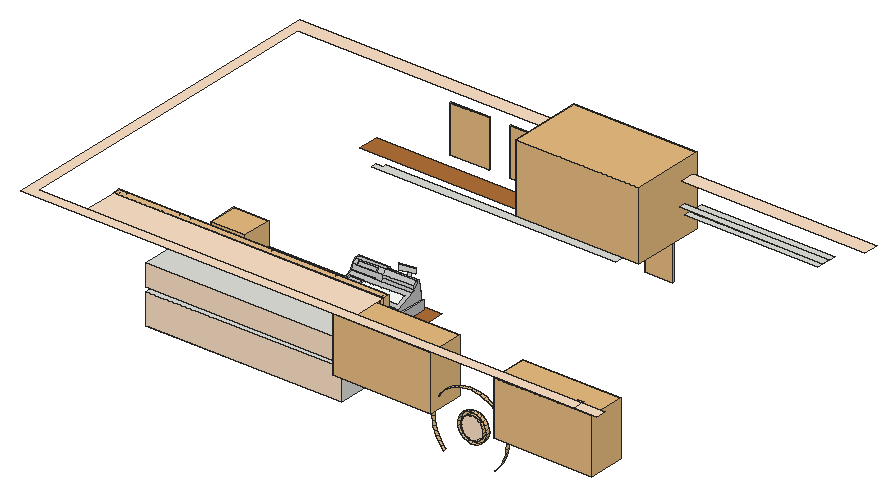
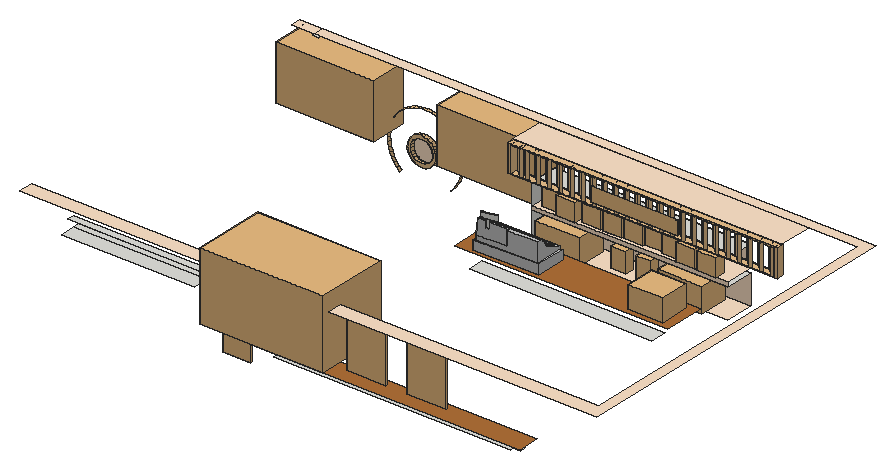
# SketchUp Ruby script. Lengths in inches.
U = 1.inch
M = Sketchup.active_model
def pt(a) = Geom::Point3d.new(a.map { |v| v * U })
def face(e, loops, mat)
  f = e.add_face(loops[0].map { |a| pt(a) })
  loops[1..].each { |l| e.add_face(l.map { |a| pt(a) }).erase! }
  f.material = f.back_material = mat if mat
  f
end
# faces: each face lists its corners as indices into pts; further lists are holes
def faces(e, pts, list, mat = nil) = list.each { |f| face(e, (f[0].is_a?(Array) ? f : [f]).map { |l| l.map { |i| pts[i] } }, mat) }
# xy, xz, yz: faces in a plane at the given z, y or x. An outline is a flat list of corners, or four numbers for a rectangle; further outlines are holes
def ring(l) = l.size == 4 ? [[l[0], l[1]], [l[2], l[1]], [l[2], l[3]], [l[0], l[3]]] : l.each_slice(2).to_a
def flat(e, list, mat, &to3) = list.each { |f| face(e, (f[0].is_a?(Array) ? f : [f]).map { |l| ring(l).map { |u, v| to3.(u, v) } }, mat) }
def xy(e, z, list, mat = nil) = flat(e, list, mat) { |x, y| [x, y, z] }
def xz(e, y, list, mat = nil) = flat(e, list, mat) { |x, z| [x, y, z] }
def yz(e, x, list, mat = nil) = flat(e, list, mat) { |y, z| [x, y, z] }
def lines(e, pts, list) = list.each { |a, b| e.add_line(pt(pts[a]), pt(pts[b])) }
# prism: a flat outline (further loops are holes) pulled along v
def prism(e, loops, v, mat = nil)
  f = face(e, loops, mat); d = Geom::Vector3d.new(v.map { |x| x * U })
  f.pushpull(f.normal.samedirection?(d) ? d.length : -d.length)
end
def box(e, o, s, mat = nil) = prism(e, [[o, [o[0] + s[0], o[1], o[2]], [o[0] + s[0], o[1] + s[1], o[2]], [o[0], o[1] + s[1], o[2]]]], [0, 0, s[2]], mat)
def at(x, y, z, deg = 0) = Geom::Transformation.translation(pt([x, y, z])) * Geom::Transformation.rotation(ORIGIN, Z_AXIS, deg.degrees)
def axes(o, x, y, z) = Geom::Transformation.new([*x, 0, *y, 0, *z, 0, *pt(o).to_a, 1])
def part(name) = M.definitions.add(name)
# library, detail: a bought-in or finely detailed component or shape, given as its bounding box
def library(name, o, s) = part(name).tap { |d| box(d.entities, o, s) }
def detail(e, o, s) = box(e.add_group.entities, o, s)
def put(e, d, t, mat = nil) = e.add_instance(d, t).tap { |i| i.material = mat if mat }
def group(e, t, mat = nil) = e.add_group.tap { |g| g.transformation = t; g.material = mat if mat }.entities
root = M.entities
M.materials.add("[Color C02]").color = [255, 228, 201]
M.materials.add("[Wood Bamboo]").color = [177, 112, 56]
M.materials.add("cash register keys").color = [249, 253, 248]
M.materials.add("ciber café cafeteira 2").color = [198, 198, 198]
M.materials.add("images").color = [235, 194, 141]
c1 = library("kitchen",[57.57,5.21,10.61],[18.31,18.31,13.72])
c2 = library("Group\#123",[0,0,0],[8.32,16.8,15.65])
c3 = library("Espresso+machine+low+poly",[-3.8125,0,0],[25.21,40.375,21.95])
c4 = library("Group\#75",[0,0,0],[34.67,0.75,41.45])
c5 = part("组\#40")
prism(c5.entities,[[[0,18.82,110.24],[218.9,18.82,110.24],[218.9,18.82,0],[0,18.82,0]],[[2.84,18.82,2.84],[216.06,18.82,2.84],[216.06,18.82,107.4],[2.84,18.82,107.4]]],[0,-18.82,0])
c6 = part("组\#36")
prism(c6.entities,[[[1.84,0,0],[0,0,0],[5.28,7.875,0],[7.11,7.875,0]]],[0,0,104.5625])
c7 = part("组\#49")
put(c7.entities,c5,at(0,1.23,0),"images")
put(c7.entities,c6,axes([8.22,1.23,2.84],[1.25286,0,0],[0,2.39,0],[0,0,1]),"images")
put(c7.entities,c6,axes([17.26,1.23,2.84],[1.25286,0,0],[0,2.39,0],[0,0,1]),"images")
put(c7.entities,c6,axes([26.3,1.23,2.84],[1.25286,0,0],[0,2.39,0],[0,0,1]),"images")
put(c7.entities,c6,axes([35.35,1.23,2.84],[1.25286,0,0],[0,2.39,0],[0,0,1]),"images")
put(c7.entities,c6,axes([71.52,1.23,2.84],[1.25286,0,0],[0,2.39,0],[0,0,1]),"images")
put(c7.entities,c6,axes([62.47,1.23,2.84],[1.25286,0,0],[0,2.39,0],[0,0,1]),"images")
put(c7.entities,c6,axes([44.39,1.23,2.84],[1.25286,0,0],[0,2.39,0],[0,0,1]),"images")
put(c7.entities,c6,axes([53.43,1.23,2.84],[1.25286,0,0],[0,2.39,0],[0,0,1]),"images")
put(c7.entities,c6,axes([89.6,1.23,2.84],[1.25286,0,0],[0,2.39,0],[0,0,1]),"images")
put(c7.entities,c6,axes([80.56,1.23,2.84],[1.25286,0,0],[0,2.39,0],[0,0,1]),"images")
put(c7.entities,c6,axes([98.64,1.23,2.84],[1.25286,0,0],[0,2.39,0],[0,0,1]),"images")
put(c7.entities,c6,axes([107.69,1.23,2.84],[1.25286,0,0],[0,2.39,0],[0,0,1]),"images")
put(c7.entities,c6,axes([125.77,1.23,2.84],[1.25286,0,0],[0,2.39,0],[0,0,1]),"images")
put(c7.entities,c6,axes([143.85,1.23,2.84],[1.25286,0,0],[0,2.39,0],[0,0,1]),"images")
put(c7.entities,c6,axes([116.73,1.23,2.84],[1.25286,0,0],[0,2.39,0],[0,0,1]),"images")
put(c7.entities,c6,axes([134.8125,1.23,2.84],[1.25286,0,0],[0,2.39,0],[0,0,1]),"images")
put(c7.entities,c6,axes([180.02,1.23,2.84],[1.25286,0,0],[0,2.39,0],[0,0,1]),"images")
put(c7.entities,c6,axes([170.98,1.23,2.84],[1.25286,0,0],[0,2.39,0],[0,0,1]),"images")
put(c7.entities,c6,axes([152.9,1.23,2.84],[1.25286,0,0],[0,2.39,0],[0,0,1]),"images")
put(c7.entities,c6,axes([161.9375,1.23,2.84],[1.25286,0,0],[0,2.39,0],[0,0,1]),"images")
put(c7.entities,c6,axes([198.11,1.23,2.84],[1.25286,0,0],[0,2.39,0],[0,0,1]),"images")
put(c7.entities,c6,axes([189.07,1.23,2.84],[1.25286,0,0],[0,2.39,0],[0,0,1]),"images")
put(c7.entities,c6,axes([207.15,1.23,2.84],[1.25286,0,0],[0,2.39,0],[0,0,1]),"images")
put(c7.entities,c6,axes([3.02,1.23,2.84],[1.25286,0,0],[0,2.39,0],[0,0,1]),"images")
c8 = library("ME COFFCE",[24.16,0,0],[47.26,9.94,0.98])
c9 = library("Countertop blender",[-3.14,-3.14,0],[6.83,6.28,15])
c10 = part("Component\#80")
xy(c10.entities,0,[[4.632,0.029,4.499,0.032,4.417,0.044,4.351,0.06,4.27,0.071,4.201,0.069,4.158,0.068,4.114,0.081,4.08,0.096,4.058,0.095,4.037,0.097,4.036,0.106,4.019,0.112,3.989,0.137,3.907,0.15,3.851,0.172,3.794,0.2,3.729,0.203,3.682,0.236,3.678,0.265,3.623,0.28,3.603,0.307,3.598,0.343,3.568,0.367,3.529,0.378,3.516,0.396,3.507,0.423,3.511,0.432,3.533,0.433,3.574,0.441,3.616,0.451,3.62,0.461,3.608,0.47,3.587,0.469,3.565,0.471,3.547,0.486,3.546,0.495,3.537,0.562,3.538,0.589,3.589,0.609,3.579,0.646,3.514,0.649,3.375,0.645,3.369,0.654,3.389,0.659,3.403,0.676,3.44,0.684,3.438,0.693,3.42,0.708,3.408,0.717,3.387,0.717,3.365,0.721,3.363,0.732,3.367,0.742,3.517,0.746,3.538,0.751,3.516,0.753,3.495,0.752,3.486,0.779,3.497,0.819,3.504,0.84,3.526,0.841,3.54,0.857,3.528,0.866,3.506,0.866,3.441,0.873,3.397,0.876,3.373,0.894,3.309,0.897,3.261,0.893,3.262,0.884,3.259,0.866,3.238,0.865,3.083,0.856,3.035,0.855,3.008,0.852,3.01,0.843,3.014,0.81,3.027,0.792,3.071,0.789,3.08,0.759,3.04,0.705,3.038,0.638,3.019,0.621,3.032,0.603,3.047,0.576,3.014,0.54,2.974,0.519,2.841,0.478,2.675,0.437,2.623,0.431,2.62,0.412,2.613,0.385,2.616,0.366,2.617,0.355,2.596,0.352,2.528,0.343,2.51,0.285,2.445,0.254,2.376,0.252,2.205,0.247,2.168,0.21,2.132,0.202,2.11,0.201,2.053,0.19,1.984,0.189,1.955,0.201,1.979,0.218,2.018,0.244,2.061,0.278,2.112,0.3,2.26,0.308,2.267,0.336,2.266,0.345,2.286,0.35,2.301,0.358,2.315,0.376,2.276,0.384,2.267,0.412,2.265,0.421,2.286,0.424,2.334,0.425,2.348,0.442,2.347,0.451,2.36,0.472,2.39,0.486,2.454,0.488,2.439,0.515,2.421,0.531,2.398,0.537,2.355,0.543,2.335,0.563,2.285,0.578,2.254,0.644,2.248,0.683,2.182,0.693,2.126,0.712,2.061,0.712,2.007,0.718,1.977,0.735,1.989,0.763,1.98,0.828,1.916,0.859,1.855,0.871,1.846,0.928,1.782,0.964,1.711,0.971,1.708,0.99,1.664,0.995,1.588,1,1.432,0.996,1.405,0.995,1.407,0.986,1.408,0.977,1.386,0.948,1.391,0.911,1.341,0.889,1.325,0.821,1.33,0.784,1.308,0.756,1.253,0.731,1.246,0.701,1.193,0.633,1.181,0.607,1.145,0.595,1.083,0.581,0.919,0.563,0.876,0.562,0.894,0.555,0.897,0.535,0.918,0.535,0.94,0.531,0.942,0.522,0.923,0.506,0.867,0.486,0.848,0.469,0.827,0.466,0.829,0.455,0.835,0.418,0.87,0.403,0.867,0.384,0.83,0.351,0.816,0.335,0.818,0.326,0.823,0.291,0.826,0.271,0.828,0.26,0.808,0.254,0.744,0.253,0.573,0.248,0.488,0.246,0.425,0.237,0.341,0.196,0.294,0.19,0.298,0.162,0.303,0.131,0.287,0.103,0.194,0.082,0.131,0.073,0.061,0.078,0.013,0.077,0,0.094,0,0.215,0.054,0.209,0.124,0.23,0.173,0.258,0.203,0.264,0.218,0.266,0.221,0.273,0.249,0.292,0.279,0.299,0.322,0.32,0.363,0.33,0.38,0.34,0.378,0.387,0.4,0.399,0.434,0.393,0.463,0.402,0.514,0.423,0.56,0.425,0.566,0.438,0.569,0.466,0.563,0.49,0.59,0.48,0.621,0.481,0.687,0.483,0.767,0.49,0.774,0.517,0.769,0.552,0.767,0.565,0.776,0.577,0.807,0.605,0.85,0.626,0.895,0.639,0.893,0.652,0.89,0.667,0.9,0.679,0.951,0.7,0.966,0.726,1.029,0.751,1.059,0.757,1.069,0.769,1.067,0.782,1.084,0.794,1.106,0.807,1.104,0.82,1.094,0.88,1.092,0.894,1.058,0.895,1.113,0.908,1.175,0.909,1.222,0.911,1.224,0.924,1.227,0.953,1.245,0.963,1.28,0.964,1.272,0.993,1.231,1.007,1.232,1.02,1.231,1.029,1.246,1.032,1.277,1.037,1.343,1.039,1.354,1.044,1.345,1.05,1.317,1.055,1.295,1.073,1.293,1.086,1.277,1.113,1.22,1.14,1.231,1.159,1.231,1.195,1.484,1.207,1.592,1.192,1.643,1.172,1.703,1.165,1.792,1.138,1.84,1.137,1.864,1.121,1.922,1.089,2.01,1.068,2.021,1.028,2.104,1.005,2.192,0.984,2.245,0.952,2.308,0.917,2.33,0.877,2.413,0.852,2.471,0.821,2.476,0.783,2.544,0.758,2.58,0.725,2.618,0.675,2.744,0.708,2.739,0.745,2.769,0.757,2.767,0.776,2.735,0.793,2.805,0.85,2.85,0.833,2.914,0.838,2.988,0.881,3.03,0.892,3.049,0.911,3.09,0.921,3.089,0.93,3.089,0.967,3.146,0.985,3.191,1.007,3.22,1.034,3.234,1.05,3.207,1.081,3.261,1.105,3.284,1.08,3.37,1.08,3.383,1.061,3.404,1.062,3.496,1.065,3.538,1.073,3.536,1.082,3.512,1.1,3.491,1.102,3.465,1.131,3.372,1.149,3.433,1.171,3.499,1.16,3.52,1.163,3.599,1.177,3.663,1.183,3.6875,1.2,3.731,1.201,3.762,1.207,3.76,1.225,3.79,1.24,3.812,1.238,3.882,1.24,3.968,1.24,3.998,1.213,4.009,1.172,3.973,1.161,3.951,1.161,3.801,1.154,3.775,1.154,3.765,1.144,3.766,1.135,3.77,1.105,3.777,1.096,3.798,1.096,3.841,1.097,3.863,1.093,3.865,1.084,3.866,1.07,3.858,1.049,3.816,1.046,3.795,1.04,3.807,1.031,3.808,1.022,3.776,0.942,3.706,0.938,3.721,0.911,3.764,0.912,3.771,0.894,3.759,0.866,3.755,0.856,3.734,0.853,3.691,0.85,3.689,0.822,3.757,0.801,3.76,0.773,3.751,0.764,3.73,0.763,3.709,0.758,3.71,0.749,3.731,0.749,3.748,0.743,3.721,0.705,3.722,0.696,3.744,0.697,3.765,0.695,3.774,0.631,3.777,0.608,3.778,0.598,3.757,0.596,3.693,0.591,3.646,0.588,3.647,0.579,3.667,0.552,3.748,0.54,3.752,0.513,3.738,0.496,3.723,0.489,3.735,0.48,3.739,0.448,3.741,0.439,3.762,0.439,3.805,0.438,3.875,0.433,3.873,0.406,3.854,0.387,3.833,0.384,3.791,0.383,3.77,0.38,3.771,0.371,3.814,0.367,3.826,0.359,3.829,0.34,3.857,0.327,3.927,0.327,3.955,0.314,3.962,0.303,3.983,0.303,4.049,0.291,4.084,0.267,4.093,0.238,4.127,0.225,4.17,0.226,4.213,0.22,4.214,0.211,4.205,0.202,4.183,0.201,4.17,0.185,4.171,0.174,4.193,0.17,4.21,0.163,4.236,0.125,4.244,0.107,4.265,0.11,4.392,0.116,4.482,0.121,4.522,0.099,4.607,0.101,4.644,0.109,4.658,0.119,4.743,0.123,4.792,0.12,4.803,0.111,4.942,0.113,4.96,0.097,4.962,0.079,4.955,0.052,4.866,0.036,4.802,0.034],[7.489,0.131,7.472,0.169,7.381,0.18,7.377,0.199,7.376,0.209,7.353,0.211,7.309,0.209,7.251,0.188,7.144,0.235,7.104,0.241,7.082,0.24,7.037,0.239,6.97,0.244,6.939,0.263,6.891,0.285,6.888,0.304,6.875,0.323,6.852,0.322,6.807,0.326,6.797,0.354,6.778,0.37,6.733,0.374,6.726,0.383,6.723,0.402,6.721,0.455,6.717,0.483,6.721,0.493,6.743,0.493,6.787,0.497,6.786,0.507,6.785,0.516,6.762,0.518,6.727,0.529,6.725,0.538,6.723,0.557,6.714,0.617,6.706,0.672,6.713,0.701,6.75,0.712,6.794,0.72,6.792,0.73,6.806,0.749,6.837,0.767,6.86,0.768,6.868,0.785,6.849,0.801,6.826,0.803,6.782,0.801,6.718,0.817,6.699,0.833,6.703,0.843,6.725,0.846,6.747,0.851,6.783,0.867,6.787,0.92,6.771,0.95,6.746,0.967,6.677,0.979,6.627,0.978,6.493,0.974,6.465,0.971,6.467,0.961,6.468,0.952,6.471,0.93,6.423,0.912,6.426,0.893,6.398,0.858,6.348,0.852,6.304,0.848,6.305,0.839,6.308,0.82,6.305,0.769,6.29,0.718,6.293,0.699,6.277,0.691,6.233,0.685,6.238,0.657,6.245,0.647,6.267,0.648,6.312,0.647,6.314,0.637,6.316,0.618,6.314,0.596,6.293,0.591,6.271,0.586,6.272,0.576,6.28,0.526,6.272,0.471,6.166,0.43,6.055,0.424,6.0625,0.415,6.085,0.415,6.107,0.416,6.152,0.413,6.151,0.384,6.131,0.367,6.061,0.35,6.031,0.326,5.93,0.294,5.916,0.277,5.918,0.268,5.886,0.255,5.764,0.251,5.697,0.25,5.659,0.241,5.65,0.229,5.628,0.229,5.6,0.228,5.545,0.226,5.433,0.226,5.311,0.225,5.247,0.237,5.222,0.253,5.19,0.283,5.149,0.292,4.999,0.29,4.947,0.296,4.93,0.302,4.889,0.313,4.817,0.311,4.776,0.317,4.768,0.367,4.705,0.408,4.717,0.44,4.76,0.448,4.774,0.465,4.773,0.475,4.77,0.494,4.765,0.522,4.719,0.531,4.711,0.578,4.694,0.679,4.723,0.706,4.722,0.716,4.699,0.717,4.694,0.746,4.738,0.752,4.733,0.786,4.726,0.795,4.703,0.794,4.681,0.794,4.679,0.803,4.678,0.813,4.679,0.837,4.919,0.849,5.039,0.835,5.075,0.822,5.092,0.815,5.048,0.814,5.003,0.8125,4.962,0.79,4.948,0.772,4.95,0.763,4.912,0.752,4.89,0.749,4.892,0.74,4.896,0.711,4.898,0.701,4.921,0.7,4.993,0.702,5.038,0.703,5.06,0.703,5.073,0.694,5.059,0.677,5.001,0.656,4.89,0.646,4.868,0.645,4.869,0.636,4.874,0.607,4.982,0.596,4.979,0.545,5.01,0.529,5.073,0.521,5.081,0.474,5.056,0.454,5.046,0.444,5.024,0.443,4.979,0.442,4.957,0.442,4.938,0.42,4.952,0.372,4.96,0.353,5.045,0.351,5.156,0.354,5.191,0.341,5.193,0.331,5.195,0.322,5.218,0.317,5.249,0.333,5.307,0.349,5.424,0.352,5.501,0.328,5.545,0.329,5.567,0.329,5.598,0.349,5.64,0.365,5.706,0.369,5.818,0.372,5.855,0.38,5.851,0.411,5.836,0.43,5.814,0.432,5.816,0.451,5.858,0.505,5.959,0.539,5.952,0.584,5.949,0.608,5.972,0.635,6.016,0.641,6.039,0.642,6.03,0.661,6.027,0.68,6.026,0.689,5.981,0.69,5.958,0.69,5.951,0.699,5.95,0.709,5.948,0.718,6.014,0.727,6.018,0.737,5.973,0.743,5.964,0.764,5.982,0.794,5.956,0.848,6.057,0.854,6.095,0.862,6.124,0.889,6.172,0.903,6.149,0.907,6.105,0.906,6.04,0.923,6.013,1.031,6.003,1.055,5.991,1.064,6.041,1.068,6.164,1.071,6.253,1.071,6.3,1.063,6.321,1.035,6.322,1.025,6.351,1.023,6.434,1.026,6.569,1.029,6.692,1.033,6.742,1.034,6.772,1.062,7.018,1.068,7.114,1.064,7.159,1.065,7.163,1.036,7.142,0.987,7.149,0.939,7.105,0.928,7.083,0.925,7.069,0.906,7.02,0.856,7.001,0.839,7.005,0.81,7.012,0.76,6.99,0.718,6.98,0.67,6.983,0.649,6.985,0.639,6.97,0.622,6.939,0.607,6.927,0.578,6.935,0.556,6.953,0.55,6.945,0.528,6.924,0.482,6.939,0.379,7.004,0.35,7.007,0.331,7.009,0.322,7.039,0.306,7.171,0.281,7.315,0.283,7.338,0.283,7.35,0.274,7.354,0.245,7.394,0.239,7.466,0.244,7.585,0.266,7.626,0.258,7.644,0.249,7.651,0.239,7.679,0.238,7.898,0.265,8.014,0.269,8.064,0.27,8.092,0.271,8.114,0.271,8.119,0.281,8.112,0.328,8.11,0.347,8.089,0.378,8.058,0.396,8.043,0.424,8.036,0.474,8.031,0.515,7.975,0.554,7.967,0.613,8.004,0.67,8.119,0.687,8.117,0.706,8.115,0.716,8.12,0.726,8.147,0.726,8.263,0.742,8.307,0.748,8.359,0.773,8.403,0.779,8.426,0.78,8.436,0.79,8.473,0.803,8.539,0.809,8.648,0.834,8.668,0.854,8.738,0.872,8.776,0.888,8.859,0.89,8.993,0.896,9.124,0.878,9.175,0.877,9.218,0.847,9.27,0.832,9.315,0.833,9.346,0.848,9.413,0.85,9.525,0.853,9.57,0.852,9.633,0.84,9.635,0.82,9.569,0.811,9.453,0.799,9.409,0.797,9.462,0.77,9.503,0.759,9.571,0.754,9.593,0.754,9.605,0.745,9.608,0.726,9.696,0.69,9.698,0.671,9.673,0.644,9.629,0.638,9.627,0.609,9.684,0.606,9.717,0.607,9.739,0.607,9.735,0.598,9.663,0.546,9.641,0.54,9.643,0.531,9.665,0.531,9.673,0.512,9.569,0.495,9.57,0.443,9.555,0.423,9.49,0.407,9.44,0.406,9.418,0.405,9.396,0.407,9.391,0.397,9.394,0.378,9.466,0.38,9.488,0.381,9.495,0.371,9.442,0.346,9.332,0.334,9.318,0.316,9.316,0.288,9.311,0.238,9.303,0.222,9.28,0.221,9.203,0.219,9.076,0.211,8.826,0.204,8.743,0.201,8.698,0.203,8.685,0.212,8.655,0.23,8.627,0.232,8.582,0.23,8.51,0.228,8.47,0.234,8.468,0.244,8.454,0.263,8.432,0.262,8.388,0.261,8.138,0.252,8.143,0.223,8.091,0.198,7.983,0.176,7.937,0.153,7.865,0.151,7.748,0.148],[9.141,1.006,9.078,1.05,9.072,1.088,9.069,1.108,9.089,1.125,9.177,1.135,9.171,1.137,9.231,1.151,9.227,1.172,9.231,1.182,9.254,1.183,9.298,1.184,9.347,1.164,9.397,1.165,9.504,1.161,9.571,1.167,9.608,1.181,9.647,1.223,9.712,1.237,9.726,1.257,9.75,1.279,9.795,1.28,9.907,1.283,9.963,1.285,9.96,1.304,9.956,1.333,9.966,1.343,9.988,1.344,10.082,1.351,10.2,1.357,10.223,1.355,10.224,1.345,10.227,1.326,10.238,1.288,10.207,1.272,10.163,1.264,10.046,1.258,10.019,1.253,10.02,1.243,10.006,1.223,9.94,1.216,9.913,1.211,9.914,1.201,9.858,1.161,9.768,1.129,9.73,1.116,9.686,1.115,9.558,1.104,9.489,1.081,9.366,1.077,9.322,1.069,9.325,1.049,9.296,1.022,9.247,1.011],[4.831,1.075,4.757,1.083,4.65,1.119,4.613,1.135,4.625,1.167,4.627,1.186,4.662,1.214,4.673,1.216,4.762,1.221,4.878,1.237,4.9,1.237,4.91,1.247,4.982,1.254,5.105,1.257,5.163,1.252,5.182,1.235,5.185,1.216,5.253,1.215,5.293,1.209,5.326,1.181,5.282,1.175,5.259,1.174,5.221,1.166,5.222,1.125,5.197,1.105,5.125,1.098,5.009,1.085,4.876,1.077]])
p = [[0,0,0],[0,0.094,0]]
lines(c10.entities,p,[[0,1]])
c11 = part("PointCash_Register")
g1 = group(c11.entities,at(0,-0.25,0))
xy(g1,0,[[0,0.25,16,16.25]],"ciber café cafeteira 2")
xy(g1,4,[[[0,0.25,16,16.25],[0.5,0.75,15.5,15.75]]],"ciber café cafeteira 2")
xz(g1,0.25,[[[0,0,16,4],[0.5,0.5,15.5,3.5]],[0.5,0.5,15.5,3.5]],"ciber café cafeteira 2")
xz(g1,0.75,[[0.5,4,15.5,5.4]],"ciber café cafeteira 2")
xz(g1,15.75,[[0.5,4,0.5,12,8,12,8,6.03,15.5,6.03,15.5,4]],"ciber café cafeteira 2")
xz(g1,16.25,[[0,0,16,4]],"ciber café cafeteira 2")
yz(g1,0,[[0.25,0,16.25,4]],"ciber café cafeteira 2")
yz(g1,0.5,[[0.75,4,0.75,5.4,10.3,8.38,12.13,7.58,12.28,7.93,10.45,8.73,11.27,10.62,13.31,11.97,15.75,12,15.75,4]],"ciber café cafeteira 2")
yz(g1,1.2,[[2.29,5.36,8.02,7.14,7.87,7.62,2.14,5.83]],"ciber café cafeteira 2")
yz(g1,1.5,[[11.6875,9.99,12.73,11.58,11.27,10.62]],"ciber café cafeteira 2")
yz(g1,4.2,[[2.29,5.36,2.14,5.83,7.87,7.62,8.02,7.14]],"ciber café cafeteira 2")
yz(g1,6.25,[[12.13,7.58,10.3,8.38,10.45,8.73,12.28,7.93],[11.6875,9.99,11.27,10.62,12.73,11.58]],"ciber café cafeteira 2")
yz(g1,8,[[15.75,6.03,15.75,12,14.72,11.99]],"ciber café cafeteira 2")
yz(g1,15.5,[[0.75,4,15.75,4,15.75,6.03,14.72,11.99,13.31,11.97,13.75,11.07,11.46,9.17,10.78,9.5,10.3,8.38,0.75,5.4],[11.46,9.17,13.75,11.07,13.31,11.97,11.27,10.62,10.78,9.5]],"ciber café cafeteira 2")
yz(g1,16,[[0.25,0,16.25,4]],"ciber café cafeteira 2")
p = [[15.5,0.75,5.4],[15.5,10.3,8.38],[8,10.3,8.38],[6.25,10.3,8.38],[0.5,10.3,8.38],[0.5,0.75,5.4],
  [4.5625,2.43,5.92],[4.5625,7.68,7.5625],[14.5625,7.68,7.5625],[14.5625,2.43,5.92],[1.2,2.14,5.83],[1.2,7.87,7.62],
  [4.2,7.87,7.62],[4.2,2.14,5.83],[4.2,2.29,5.36],[1.2,2.29,5.36],[1.2,8.02,7.14],[4.2,8.02,7.14],
  [15.5,14.72,11.99],[15.5,15.75,6.03],[8,15.75,6.03],[8,14.72,11.99],[6.25,12.13,7.58],[0.5,12.13,7.58],
  [6.25,12.28,7.93],[0.5,12.28,7.93],[6.25,10.45,8.73],[0.5,10.45,8.73],[0.5,11.27,10.62],[8,10.78,9.5],
  [8,11.27,10.62],[6.25,11.27,10.62],[1.5,11.27,10.62],[15.5,10.78,9.5],[15.5,11.27,10.62],[6.25,11.6875,9.99],
  [1.5,11.6875,9.99],[6.25,12.73,11.58],[1.5,12.73,11.58],[8,13.31,11.97],[0.5,13.31,11.97],[15.5,13.31,11.97],
  [8,15.75,12],[0.5,15.75,12]]
faces(g1,p,[[[0,1,2,3,4,5],[6,7,8,9],[10,11,12,13]],[10,13,14,15],[16,15,14,17],[18,19,20,21],[12,11,16,17],[4,3,22,23],[23,22,24,25],[26,27,25,24],
  [28,27,26,3,2,29,30,31,32],[1,33,29,2],[30,29,33,34],[32,31,35,36],[35,37,38,36],[31,30,39,40,28,32,38,37],[41,39,30,34],[40,39,21,42,43],
  [18,21,39,41]],"ciber café cafeteira 2")
faces(g1,p,[[7,6,9,8]],"cash register keys")
g2 = group(g1,at(10.92,13.68,9.01,20))
xy(g2,0,[[2,0,2,0.87,2.75,0.43]])
xy(g2,4.5,[[0,0,2,0.5],[2,0,2.75,0.43,2,0.87,2,0.5,4,0.5,4,0],[2,0,2.75,0.43,2,0.87],[0,0.5,4,1]])
xy(g2,6.5,[[0,0,4,0.5],[0,0.5,4,1]])
xz(g2,0,[[0,4.5,4,6.5]])
xz(g2,1,[[0,4.5,4,6.5]])
yz(g2,0,[[0,4.5,0.5,6.5],[0.5,4.5,1,6.5]])
yz(g2,2,[[0,0,0.87,4.5]])
yz(g2,4,[[0,4.5,0.5,6.5],[0.5,4.5,1,6.5]])
p = [[2,0,0],[2.75,0.43,0],[2.75,0.43,4.5],[2,0,4.5],[2,0.87,0],[2,0.87,4.5]]
faces(g2,p,[[0,1,2,3],[1,4,5,2]])
c12 = library("suspension plantes",[-8.73,-11.75,0],[87.64,63.68,60.73])
c13 = library("Umbra+Bolo (1)",[-7.04,-1.89,-4.93],[32.14,86.7,48.29])
c14 = library("组件\#16",[0,0,0],[25.91,1.13,79.84])
xy(root,42.97,[[275.2,13.5,448.07,38.75]],"[Color C02]")
xy(root,49.79,[[264.58,276.18,264.58,281.06,270.96,281.06,270.96,283.81,480.22,283.81,480.22,276.18]])
xy(root,57.71,[[281.8,100.22,442.97,113.97]])
xy(root,60.5625,[[253.81,276.18,490.99,295.25]],"[Wood Bamboo]")
xy(root,69.78,[[275.2,13.5,448.07,38.75]])
xy(root,71.375,[[268.13,77.03,456.63,113.97]],"[Wood Bamboo]")
xy(root,73.09,[[275.2,13.5,448.07,38.75]],"[Color C02]")
xy(root,92.25,[[275.2,13.5,448.07,38.75]])
xy(root,98.63,[[530.43,289.72,647.93,295.72],[530.43,295.72,647.93,308.75]])
xy(root,103.32,[[525.75,289.72,652.62,295.72]])
xy(root,120,[[659.13,9,664.13,11]])
xy(root,120,[[174.82,0,664.13,0,664.13,9,183.82,9,183.82,295.72,684.57,295.72,684.57,308.75,174.82,308.75],[664.13,0,684.57,9],[227.2,9,464.82,38.75]],"[Color C02]")
xz(root,11.5,[[[564.29,54.41,561.76,54.9375,559.45,56.1,557.52,57.82,556.1,59.99,555.29,62.45,555.14,65.03,555.67,67.5625,556.83,69.87,558.56,71.8,560.72,73.22,563.18,74.03,565.76,74.18,568.29,73.65,570.6,72.49,572.53,70.76,573.95,68.6,574.76,66.14,574.91,63.56,574.38,61.03,573.22,58.71,571.49,56.78,569.33,55.37,566.87,54.56],[564.31,54.7,566.82,54.84,569.2,55.625,571.31,57,572.98,58.875,574.11,61.12,574.62,63.58,574.48,66.09,573.69,68.47,572.32,70.58,570.44,72.25,568.2,73.38,565.74,73.89,563.23,73.75,560.84,72.96,558.74,71.59,557.07,69.71,555.9375,67.47,555.43,65.01,555.57,62.5,556.35,60.11,557.73,58.01,559.61,56.34,561.85,55.21]]])
xz(root,11.5,[[564.31,54.7,561.85,55.21,559.61,56.34,557.73,58.01,556.35,60.11,555.57,62.5,555.43,65.01,555.9375,67.47,557.07,69.71,558.74,71.59,560.84,72.96,563.23,73.75,565.74,73.89,568.2,73.38,570.44,72.25,572.32,70.58,573.69,68.47,574.48,66.09,574.62,63.58,574.11,61.12,572.98,58.875,571.31,57,569.2,55.625,566.82,54.84]],"[Color C02]")
xz(root,13.5,[[275.2,42.97,448.07,69.78],[275.2,73.09,448.07,92.25]],"[Color C02]")
xz(root,14.75,[[[564.08,51.67,560.85,52.35,557.9,53.83,555.44,56.03,553.625,58.8,552.59,61.93,552.4,65.23,553.08,68.47,554.5625,71.42,556.76,73.88,559.53,75.69,562.66,76.73,565.96,76.91,569.2,76.24,572.15,74.75,574.61,72.55,576.42,69.79,577.46,66.65,577.65,63.35,576.97,60.12,575.48,57.17,573.28,54.7,570.52,52.89,567.38,51.86],[564.29,54.41,566.87,54.56,569.33,55.37,571.49,56.78,573.22,58.71,574.38,61.03,574.91,63.56,574.76,66.14,573.95,68.6,572.53,70.76,570.6,72.49,568.29,73.65,565.76,74.18,563.18,74.03,560.72,73.22,558.56,71.8,556.83,69.87,555.67,67.5625,555.14,65.03,555.29,62.45,556.1,59.99,557.52,57.82,559.45,56.1,561.76,54.9375]]],"images")
xz(root,38.75,[[275.2,69.78,448.07,73.09]],"[Color C02]")
yz(root,448.07,[[13.5,42.97,38.75,69.78],[13.5,73.09,38.75,92.25]])
p = [[589.71,9,42.0625],[587.09,9,39.29],[587.09,11.5,39.29],[589.71,11.5,42.0625],[542.05,9,39.4],[539.44,9,42.18],
  [539.44,11.5,42.18],[542.05,11.5,39.4],[592,9,45.12],[592,11.5,45.12],[537.17,9,45.25],[537.17,11.5,45.25],
  [593.91,9,48.42],[593.91,11.5,48.42],[535.27,9,48.56],[535.27,11.5,48.56],[595.43,9,51.92],[595.43,11.5,51.92],
  [533.77,9,52.06],[533.77,11.5,52.06],[564.08,11.5,51.67],[560.85,11.5,52.35],[560.85,14.75,52.35],[564.08,14.75,51.67],
  [567.38,11.5,51.86],[567.38,14.75,51.86],[596.54,9,55.57],[596.54,11.5,55.57],[570.52,11.5,52.89],[570.52,14.75,52.89],
  [532.68,9,55.72],[532.68,11.5,55.72],[557.9,11.5,53.83],[557.9,14.75,53.83],[573.28,11.5,54.7],[573.28,14.75,54.7],
  [555.44,11.5,56.03],[555.44,14.75,56.03],[561.76,11.5,54.9375],[564.29,11.5,54.41],[564.29,14.75,54.41],[561.76,14.75,54.9375],
  [566.87,11.5,54.56],[566.87,14.75,54.56],[569.33,11.5,55.37],[569.33,14.75,55.37],[575.48,11.5,57.17],[575.48,14.75,57.17],
  [559.45,11.5,56.1],[559.45,14.75,56.1],[571.49,11.5,56.78],[571.49,14.75,56.78],[597.21,9,59.33],[597.21,11.5,59.33],
  [532.03,9,59.48],[532.03,11.5,59.48],[553.625,11.5,58.8],[553.625,14.75,58.8],[557.52,11.5,57.82],[557.52,14.75,57.82],
  [573.22,11.5,58.71],[573.22,14.75,58.71],[576.97,11.5,60.12],[576.97,14.75,60.12],[556.1,11.5,59.99],[556.1,14.75,59.99],
  [574.38,11.5,61.03],[574.38,14.75,61.03],[552.59,11.5,61.93],[552.59,14.75,61.93],[597.4375,9,63.14],[597.4375,11.5,63.14],
  [531.8125,9,63.29],[531.8125,11.5,63.29],[555.29,11.5,62.45],[555.29,14.75,62.45],[577.65,11.5,63.35],[577.65,14.75,63.35],
  [574.91,11.5,63.56],[574.91,14.75,63.56],[552.4,11.5,65.23],[552.4,14.75,65.23],[555.14,11.5,65.03],[555.14,14.75,65.03],
  [597.23,9,66.95],[597.23,11.5,66.95],[532.04,9,67.1],[532.04,11.5,67.1],[577.46,11.5,66.65],[577.46,14.75,66.65],
  [574.76,11.5,66.14],[574.76,14.75,66.14],[555.67,11.5,67.5625],[555.67,14.75,67.5625],[553.08,11.5,68.47],[553.08,14.75,68.47],
  [573.95,11.5,68.6],[573.95,14.75,68.6],[576.42,11.5,69.79],[576.42,14.75,69.79],[596.57,9,70.71],[596.57,11.5,70.71],
  [532.72,9,70.86],[532.72,11.5,70.86],[556.83,11.5,69.87],[556.83,14.75,69.87],[554.5625,11.5,71.42],[554.5625,14.75,71.42],
  [572.53,11.5,70.76],[572.53,14.75,70.76],[574.61,11.5,72.55],[574.61,14.75,72.55],[558.56,11.5,71.8],[558.56,14.75,71.8],
  [595.49,9,74.36],[595.49,11.5,74.36],[570.6,11.5,72.49],[570.6,14.75,72.49],[533.82,9,74.51],[533.82,11.5,74.51],
  [556.76,11.5,73.88],[556.76,14.75,73.88],[560.72,11.5,73.22],[560.72,14.75,73.22],[568.29,11.5,73.65],[568.29,14.75,73.65],
  [572.15,11.5,74.75],[572.15,14.75,74.75],[563.18,11.5,74.03],[563.18,14.75,74.03],[565.76,11.5,74.18],[565.76,14.75,74.18],
  [559.53,11.5,75.69],[559.53,14.75,75.69],[593.98,9,77.87],[593.98,11.5,77.87],[535.34,9,78.01],[535.34,11.5,78.01],
  [569.2,11.5,76.24],[569.2,14.75,76.24],[562.66,11.5,76.73],[562.66,14.75,76.73],[565.96,11.5,76.91],[565.96,14.75,76.91],
  [592.08,9,81.18],[592.08,11.5,81.18],[537.25,9,81.31],[537.25,11.5,81.31],[589.8125,9,84.25],[589.8125,11.5,84.25],
  [539.54,9,84.37],[539.54,11.5,84.37],[587.2,9,87.03],[587.2,11.5,87.03],[542.17,9,87.13],[542.17,11.5,87.13],
  [584.28,9,89.49],[584.28,11.5,89.49],[545.09,9,89.58],[545.09,11.5,89.58],[581.1,9,91.59],[581.1,11.5,91.59],
  [548.29,9,91.67],[548.29,11.5,91.67],[577.69,9,93.3125],[577.69,11.5,93.3125],[551.7,9,93.375],[551.7,11.5,93.375],
  [574.11,9,94.625],[574.11,11.5,94.625],[555.29,9,94.67],[555.29,11.5,94.67],[570.4,9,95.51],[570.4,11.5,95.51],
  [559,9,95.54],[559,11.5,95.54],[562.8,9,95.98],[562.8,11.5,95.98],[566.61,9,95.97],[566.61,11.5,95.97],
  [372.1,295.21,74.82],[372.1,295.21,74.87],[385.46,295.21,72.85],[385.46,295.21,72.83]]
faces(root,p,[[0,1,2,3],[4,5,6,7],[8,0,3,9],[5,10,11,6],[12,8,9,13],[10,14,15,11],[16,12,13,17],[14,18,19,15],
  [20,21,22,23],[24,20,23,25],[26,16,17,27],[28,24,25,29],[18,30,31,19],[21,32,33,22],[34,28,29,35],[32,36,37,33],
  [38,39,40,41],[39,42,43,40],[42,44,45,43],[46,34,35,47],[48,38,41,49],[44,50,51,45],[52,26,27,53],[30,54,55,31],
  [36,56,57,37],[58,48,49,59],[50,60,61,51],[62,46,47,63],[64,58,59,65],[60,66,67,61],[56,68,69,57],[70,52,53,71],
  [54,72,73,55],[74,64,65,75],[76,62,63,77],[66,78,79,67],[68,80,81,69],[82,74,75,83],[84,70,71,85],[72,86,87,73],
  [88,76,77,89],[78,90,91,79],[92,82,83,93],[80,94,95,81],[90,96,97,91],[98,88,89,99],[100,84,85,101],[86,102,103,87],
  [104,92,93,105],[94,106,107,95],[96,108,109,97],[110,98,99,111],[112,104,105,113],[114,100,101,115],[108,116,117,109],[102,118,119,103],
  [106,120,121,107],[122,112,113,123],[116,124,125,117],[126,110,111,127],[128,122,123,129],[124,130,131,125],[120,132,133,121],[130,128,129,131],
  [134,114,115,135],[118,136,137,119],[138,126,127,139],[132,140,141,133],[142,138,139,143],[140,142,143,141],[144,134,135,145],[136,146,147,137],
  [148,144,145,149],[146,150,151,147],[152,148,149,153],[150,154,155,151],[156,152,153,157],[154,158,159,155],[160,156,157,161],[158,162,163,159],
  [164,160,161,165],[162,166,167,163],[168,164,165,169],[166,170,171,167],[172,168,169,173],[170,174,175,171],[174,176,177,175],[178,172,173,179],
  [176,178,179,177]],"images")
lines(root,p,[[180,181],[182,183]])
detail(root,[371.7,294.82,70.03],[34.67,0.75,41.45])
put(root,c1,axes([177.71,78.5,58.42],[1.6756,0,0],[0,1.42,0],[0,0,1.42]))
put(root,c2,at(302.3,30.43,73.09,90))
put(root,c2,at(321.17,30.43,73.09,90))
put(root,c3,axes([294.28,39.18,42.97],[0,-1,0],[0.97478,0,0],[0,0,1]))
put(root,c2,at(336.43,27.0625,73.09,90))
put(root,c4,at(319.08,294.82,70.03))
put(root,c2,at(352.77,25,73.09,90))
put(root,c7,axes([464.82,38.34,95.875],[-1.09,0,0],[0,0.3293,0],[0,0,0.21885]))
put(root,c8,axes([426.04,49.79,102.67],[-1.61548,0,0],[0,0,1.25],[0,0.15625,0]))
put(root,c9,axes([354.66,27.9375,42.97],[1.91114,0,0],[0,1.19,0],[0,0,1.19]))
put(root,c2,at(370.12,27.0625,73.09,90))
put(root,c9,axes([376.97,27.9375,42.97],[1.91114,0,0],[0,1.19,0],[0,0,1.19]))
put(root,c2,at(387.99,27.0625,73.09,90))
put(root,c2,at(406.49,27.0625,73.09,90))
put(root,c10,axes([401.92,295.21,73.61],[0.32297,0,0.01071],[-0.02496,0,0.75234],[0,-0.18881,0]))
put(root,c11,axes([385.9375,82.97,71.375],[3.58809,0.06889,0],[-0.03168,1.6497,0],[0,0,2.0625]))
put(root,c2,at(426.84,30.43,73.09,90))
put(root,c3,axes([402.95,38.75,42.97],[0,-1,0],[0.97478,0,0],[0,0,1]))
put(root,c2,at(442.37,27.0625,73.09,90))
put(root,c12,axes([423.73,261.87,74.04],[1.24,0,0],[0,1,0],[0,0,1]))
put(root,c13,at(535,7.89,75.46,90))
put(root,c14,axes([496.24,288.63,42.125],[0.93587,0,0],[0,0.93587,0],[0,0,0.93587]))
put(root,c13,at(677.36,7.89,75.46,90))
